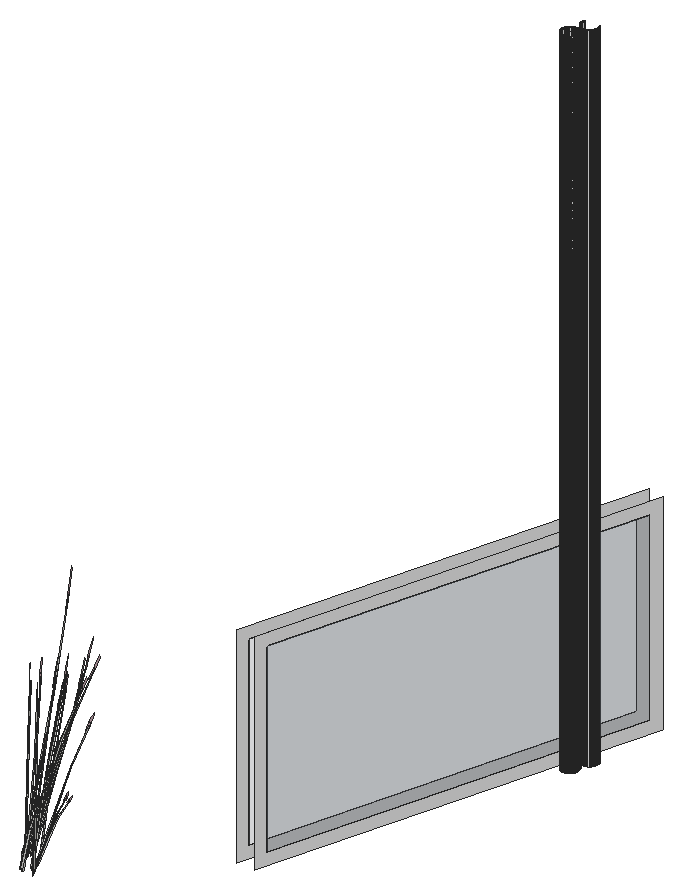
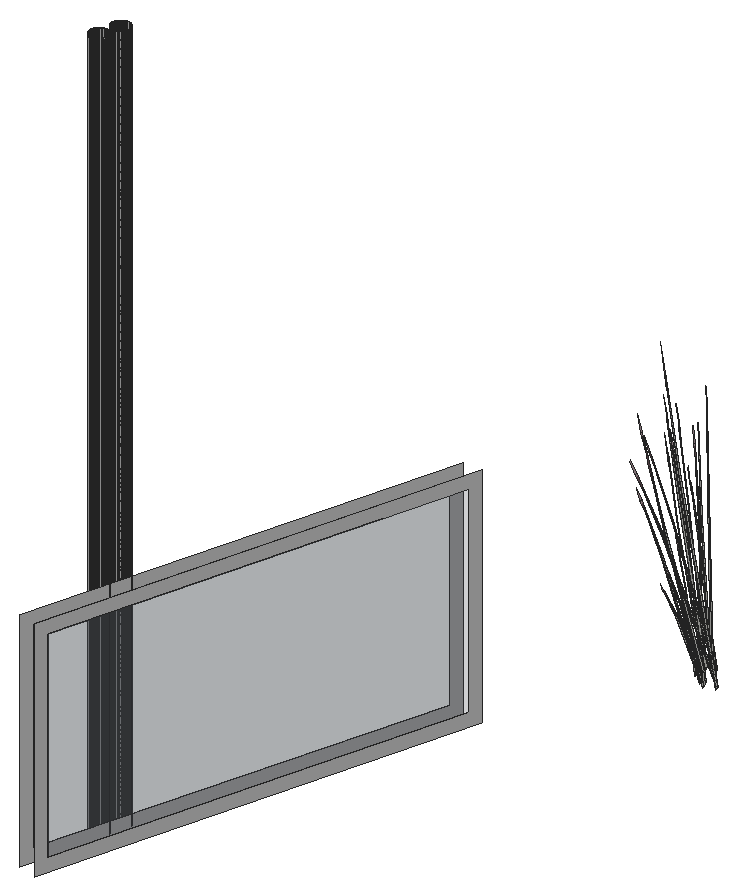
# SketchUp Ruby script. Lengths in inches.
U = 1.inch
M = Sketchup.active_model
def pt(a) = Geom::Point3d.new(a.map { |v| v * U })
def face(e, loops, mat)
  f = e.add_face(loops[0].map { |a| pt(a) })
  loops[1..].each { |l| e.add_face(l.map { |a| pt(a) }).erase! }
  f.material = f.back_material = mat if mat
  f
end
# faces: each face lists its corners as indices into pts; further lists are holes
def faces(e, pts, list, mat = nil) = list.each { |f| face(e, (f[0].is_a?(Array) ? f : [f]).map { |l| l.map { |i| pts[i] } }, mat) }
# xy, xz, yz: faces in a plane at the given z, y or x. An outline is a flat list of corners, or four numbers for a rectangle; further outlines are holes
def ring(l) = l.size == 4 ? [[l[0], l[1]], [l[2], l[1]], [l[2], l[3]], [l[0], l[3]]] : l.each_slice(2).to_a
def flat(e, list, mat, &to3) = list.each { |f| face(e, (f[0].is_a?(Array) ? f : [f]).map { |l| ring(l).map { |u, v| to3.(u, v) } }, mat) }
def xy(e, z, list, mat = nil) = flat(e, list, mat) { |x, y| [x, y, z] }
def xz(e, y, list, mat = nil) = flat(e, list, mat) { |x, z| [x, y, z] }
def yz(e, x, list, mat = nil) = flat(e, list, mat) { |y, z| [x, y, z] }
def lines(e, pts, list) = list.each { |a, b| e.add_line(pt(pts[a]), pt(pts[b])) }
# prism: a flat outline (further loops are holes) pulled along v
def prism(e, loops, v, mat = nil)
  f = face(e, loops, mat); d = Geom::Vector3d.new(v.map { |x| x * U })
  f.pushpull(f.normal.samedirection?(d) ? d.length : -d.length)
end
def box(e, o, s, mat = nil) = prism(e, [[o, [o[0] + s[0], o[1], o[2]], [o[0] + s[0], o[1] + s[1], o[2]], [o[0], o[1] + s[1], o[2]]]], [0, 0, s[2]], mat)
def at(x, y, z, deg = 0) = Geom::Transformation.translation(pt([x, y, z])) * Geom::Transformation.rotation(ORIGIN, Z_AXIS, deg.degrees)
def axes(o, x, y, z) = Geom::Transformation.new([*x, 0, *y, 0, *z, 0, *pt(o).to_a, 1])
def part(name) = M.definitions.add(name)
# library, detail: a bought-in or finely detailed component or shape, given as its bounding box
def library(name, o, s) = part(name).tap { |d| box(d.entities, o, s) }
def detail(e, o, s) = box(e.add_group.entities, o, s)
def put(e, d, t, mat = nil) = e.add_instance(d, t).tap { |i| i.material = mat if mat }
def group(e, t, mat = nil) = e.add_group.tap { |g| g.transformation = t; g.material = mat if mat }.entities
root = M.entities
M.materials.add("Glass_Basic_01").color = [105, 113, 122]
M.materials["Glass_Basic_01"].alpha = 0.25
M.materials.add("LightPink_Translucent").color = [144, 107, 117]
M.materials["LightPink_Translucent"].alpha = 0.75
M.materials.add("M01_Silver_Fog").color = [224, 224, 224]
c1 = part("blade")
p = [[2.15,0.21,22],[0,0.17,0],[0.09,0.45,0],[2.18,0.31,22],[2.29,0.31,22],[0.38,0.45,0],
  [2.48,0.24,33],[2.49,0.24,33],[2.48,0.22,33]]
faces(c1.entities,p,[[0,1,2,3],[4,5,2,3],[6,3,4,7],[8,0,3,6]])
c2 = part("seeds")
p = [[0.3,-0.1,1.38],[-0.01,-0.03,1.59],[-0.01,-0.03,0.03],[0.14,-0.07,-0.07],[0.29,-0.03,3],[0.15,0.01,3.11]]
faces(c2.entities,p,[[0,1,2,3],[1,0,4,5]],"LightPink_Translucent")
c3 = part("blade with seeds")
put(c3.entities,c1,at(0,0,0))
put(c3.entities,c2,axes([2.4,0.25,30.99],[1.5799,-0.05474,1.17369],[-0.12525,1.92788,0.29478],[-0.07173,-0.02425,1.56792]))
xz(root,421.6,[[358.82,522,358.91,636],[358.91,522,359,636]],"M01_Silver_Fog")
xz(root,421.95,[[359.74,522,359.83,636],[359.83,522,359.92,636]],"M01_Silver_Fog")
yz(root,357.51,[[420.11,522,420.2,636],[420.2,522,420.29,636]],"M01_Silver_Fog")
yz(root,358.43,[[423.26,522,423.35,636],[423.35,522,423.44,636]],"M01_Silver_Fog")
yz(root,360.31,[[420.11,522,420.2,636],[420.2,522,420.29,636]],"M01_Silver_Fog")
yz(root,361.23,[[423.26,522,423.35,636],[423.35,522,423.44,636]],"M01_Silver_Fog")
p = [[359.17,437.01,522],[340.07,371.78,522],[340.07,371.78,558],[359.17,437.01,558],[340.64,373.7,524],[358.6,435.09,524],
  [358.6,435.09,556],[340.64,373.7,556],[362.06,436.22,558],[343.2,371.78,558],[343.2,371.78,522],[362.06,436.22,522],
  [343.76,373.7,556],[361.5,434.3,556],[361.5,434.3,524],[343.76,373.7,524],[358.48,418.87,522],[358.5625,418.85,522],
  [358.5625,418.85,636],[358.48,418.87,636],[358.65,418.83,522],[358.73,418.8125,522],[358.73,418.8125,636],[358.65,418.83,636],
  [358.82,418.81,522],[358.82,418.81,636],[358.91,418.8,522],[358.91,418.8,636],[359,418.81,522],[359,418.81,636],
  [359.09,418.8125,522],[359.09,418.8125,636],[359.17,418.83,522],[359.17,418.83,636],[359.26,418.85,522],[359.26,418.85,636],
  [359.34,418.87,522],[359.34,418.87,636],[358.24,418.98,522],[358.3125,418.9375,522],[358.3125,418.9375,636],[358.24,418.98,636],
  [358.39,418.9,522],[358.39,418.9,636],[359.43,418.9,522],[359.43,418.9,636],[359.51,418.9375,522],[359.51,418.9375,636],
  [359.58,418.98,522],[359.58,418.98,636],[358.09,419.07,522],[358.16,419.02,522],[358.16,419.02,636],[358.09,419.07,636],
  [359.66,419.02,522],[359.66,419.02,636],[359.73,419.07,522],[359.73,419.07,636],[358.02,419.125,522],[358.02,419.125,636],
  [357.95,419.18,522],[357.95,419.18,636],[359.8,419.125,522],[359.8,419.125,636],[359.87,419.18,522],[359.87,419.18,636],
  [357.83,419.31,522],[357.89,419.24,522],[357.89,419.24,636],[357.83,419.31,636],[359.93,419.24,522],[359.93,419.24,636],
  [359.99,419.31,522],[359.99,419.31,636],[357.78,419.38,522],[357.78,419.38,636],[360.04,419.38,522],[360.04,419.38,636],
  [357.73,419.45,522],[357.73,419.45,636],[360.09,419.45,522],[360.09,419.45,636],[357.64,419.61,522],[357.68,419.53,522],
  [357.68,419.53,636],[357.64,419.61,636],[360.14,419.53,522],[360.14,419.53,636],[360.18,419.61,522],[360.18,419.61,636],
  [357.61,419.6875,522],[357.61,419.6875,636],[360.21,419.6875,522],[360.21,419.6875,636],[357.58,419.77,522],[357.58,419.77,636],
  [360.24,419.77,522],[360.24,419.77,636],[357.55,419.85,522],[357.55,419.85,636],[360.27,419.85,522],[360.27,419.85,636],
  [357.54,419.94,522],[357.54,419.94,636],[357.52,420.03,522],[357.52,420.03,636],[360.29,419.94,522],[360.29,419.94,636],
  [360.3,420.03,522],[360.3,420.03,636],[357.51,420.11,522],[357.51,420.11,636],[360.31,420.11,522],[360.31,420.11,636],
  [357.52,420.38,522],[357.51,420.29,522],[357.51,420.29,636],[357.52,420.38,636],[360.31,420.29,522],[360.3,420.38,522],
  [360.3,420.38,636],[360.31,420.29,636],[357.54,420.46,522],[357.54,420.46,636],[360.29,420.46,522],[360.29,420.46,636],
  [357.55,420.55,522],[357.55,420.55,636],[360.27,420.55,522],[360.27,420.55,636],[357.58,420.64,522],[357.58,420.64,636],
  [357.61,420.72,522],[357.61,420.72,636],[360.24,420.64,522],[360.24,420.64,636],[360.21,420.72,522],[360.21,420.72,636],
  [357.64,420.8,522],[357.64,420.8,636],[360.18,420.8,522],[360.18,420.8,636],[357.68,420.88,522],[357.68,420.88,636],
  [360.14,420.88,522],[360.14,420.88,636],[357.73,420.95,522],[357.73,420.95,636],[360.09,420.95,522],[360.09,420.95,636],
  [357.78,421.03,522],[357.78,421.03,636],[357.83,421.09,522],[357.83,421.09,636],[360.04,421.03,522],[360.04,421.03,636],
  [359.99,421.09,522],[359.99,421.09,636],[357.89,421.16,522],[357.89,421.16,636],[359.93,421.16,522],[359.93,421.16,636],
  [357.95,421.22,522],[357.95,421.22,636],[358.02,421.28,522],[358.02,421.28,636],[359.87,421.22,522],[359.8,421.28,522],
  [359.8,421.28,636],[359.87,421.22,636],[358.09,421.34,522],[358.09,421.34,636],[358.16,421.38,522],[358.16,421.38,636],
  [359.73,421.34,522],[359.73,421.34,636],[359.66,421.38,522],[359.66,421.38,636],[358.24,421.43,522],[358.24,421.43,636],
  [358.3125,421.47,522],[358.3125,421.47,636],[359.58,421.43,522],[359.51,421.47,522],[359.51,421.47,636],[359.58,421.43,636],
  [358.39,421.5,522],[358.39,421.5,636],[358.48,421.53,522],[358.48,421.53,636],[358.5625,421.56,522],[358.5625,421.56,636],
  [359.43,421.5,522],[359.34,421.53,522],[359.34,421.53,636],[359.43,421.5,636],[359.26,421.56,522],[359.26,421.56,636],
  [358.65,421.58,522],[358.65,421.58,636],[358.73,421.59,522],[358.73,421.59,636],[358.82,421.6,522],[358.82,421.6,636],
  [359.09,421.59,522],[359,421.6,522],[359,421.6,636],[359.09,421.59,636],[359.17,421.58,522],[359.17,421.58,636],
  [359.66,421.96,522],[359.74,421.95,522],[359.74,421.95,636],[359.66,421.96,636],[359.92,421.95,522],[360.01,421.96,522],
  [360.01,421.96,636],[359.92,421.95,636],[359.23,422.08,522],[359.32,422.05,522],[359.32,422.05,636],[359.23,422.08,636],
  [359.4,422.02,522],[359.4,422.02,636],[359.48,421.99,522],[359.48,421.99,636],[359.57,421.97,522],[359.57,421.97,636],
  [360.09,421.97,522],[360.09,421.97,636],[360.18,421.99,522],[360.18,421.99,636],[360.26,422.02,522],[360.26,422.02,636],
  [360.35,422.05,522],[360.35,422.05,636],[360.43,422.08,522],[360.43,422.08,636],[359.08,422.17,522],[359.16,422.12,522],
  [359.16,422.12,636],[359.08,422.17,636],[360.51,422.12,522],[360.51,422.12,636],[360.58,422.17,522],[360.58,422.17,636],
  [358.9375,422.27,522],[359.01,422.21,522],[359.01,422.21,636],[358.9375,422.27,636],[360.65,422.21,522],[360.65,422.21,636],
  [360.72,422.27,522],[360.72,422.27,636],[358.81,422.39,522],[358.87,422.33,522],[358.87,422.33,636],[358.81,422.39,636],
  [360.79,422.33,522],[360.79,422.33,636],[360.85,422.39,522],[360.85,422.39,636],[358.75,422.45,522],[358.75,422.45,636],
  [360.91,422.45,522],[360.91,422.45,636],[358.65,422.6,522],[358.7,422.52,522],[358.7,422.52,636],[358.65,422.6,636],
  [360.96,422.52,522],[360.96,422.52,636],[361.01,422.6,522],[361.01,422.6,636],[358.6,422.67,522],[358.6,422.67,636],
  [361.06,422.67,522],[361.06,422.67,636],[358.5625,422.75,522],[358.5625,422.75,636],[361.1,422.75,522],[361.1,422.75,636],
  [358.53,422.83,522],[358.53,422.83,636],[358.5,422.91,522],[358.5,422.91,636],[361.13,422.83,522],[361.13,422.83,636],
  [361.16,422.91,522],[361.16,422.91,636],[358.47,423,522],[358.47,423,636],[361.1875,423,522],[361.1875,423,636],
  [358.46,423.08,522],[358.46,423.08,636],[361.21,423.08,522],[361.21,423.08,636],[358.44,423.17,522],[358.44,423.17,636],
  [361.22,423.17,522],[361.22,423.17,636],[358.43,423.26,522],[358.43,423.26,636],[361.23,423.26,522],[361.23,423.26,636],
  [358.44,423.52,522],[358.43,423.44,522],[358.43,423.44,636],[358.44,423.52,636],[361.23,423.44,522],[361.22,423.52,522],
  [361.22,423.52,636],[361.23,423.44,636],[358.46,423.61,522],[358.46,423.61,636],[361.21,423.61,522],[361.21,423.61,636],
  [358.47,423.7,522],[358.47,423.7,636],[361.1875,423.7,522],[361.1875,423.7,636],[358.5,423.78,522],[358.5,423.78,636],
  [361.16,423.78,522],[361.16,423.78,636],[358.53,423.86,522],[358.53,423.86,636],[361.13,423.86,522],[361.13,423.86,636],
  [358.5625,423.94,522],[358.5625,423.94,636],[361.1,423.94,522],[361.1,423.94,636]]
faces(root,p,[[[0,1,2,3],[4,5,6,7]],[[8,9,10,11],[12,13,14,15]],[16,17,18,19],[20,21,22,23],[17,20,23,18],[21,24,25,22],[24,26,27,25],[26,28,29,27],
  [28,30,31,29],[30,32,33,31],[32,34,35,33],[34,36,37,35],[38,39,40,41],[39,42,43,40],[42,16,19,43],[36,44,45,37],
  [44,46,47,45],[46,48,49,47],[50,51,52,53],[51,38,41,52],[48,54,55,49],[54,56,57,55],[58,50,53,59],[60,58,59,61],
  [56,62,63,57],[62,64,65,63],[66,67,68,69],[67,60,61,68],[64,70,71,65],[70,72,73,71],[74,66,69,75],[72,76,77,73],
  [78,74,75,79],[76,80,81,77],[82,83,84,85],[83,78,79,84],[80,86,87,81],[86,88,89,87],[90,82,85,91],[88,92,93,89],
  [94,90,91,95],[92,96,97,93],[98,94,95,99],[96,100,101,97],[102,98,99,103],[104,102,103,105],[100,106,107,101],[106,108,109,107],
  [110,104,105,111],[108,112,113,109],[114,115,116,117],[118,119,120,121],[122,114,117,123],[119,124,125,120],[126,122,123,127],[124,128,129,125],
  [130,126,127,131],[132,130,131,133],[128,134,135,129],[134,136,137,135],[138,132,133,139],[136,140,141,137],[142,138,139,143],[140,144,145,141],
  [146,142,143,147],[144,148,149,145],[150,146,147,151],[152,150,151,153],[148,154,155,149],[154,156,157,155],[158,152,153,159],[156,160,161,157],
  [162,158,159,163],[164,162,163,165],[166,167,168,169],[160,166,169,161],[170,164,165,171],[172,170,171,173],[167,174,175,168],[174,176,177,175],
  [178,172,173,179],[180,178,179,181],[182,183,184,185],[176,182,185,177],[186,180,181,187],[188,186,187,189],[190,188,189,191],[192,193,194,195],
  [193,196,197,194],[183,192,195,184],[198,190,191,199],[200,198,199,201],[202,200,201,203],[204,205,206,207],[208,204,207,209],[196,208,209,197],
  [210,211,212,213],[214,215,216,217],[218,219,220,221],[219,222,223,220],[222,224,225,223],[224,226,227,225],[226,210,213,227],[215,228,229,216],
  [228,230,231,229],[230,232,233,231],[232,234,235,233],[234,236,237,235],[238,239,240,241],[239,218,221,240],[236,242,243,237],[242,244,245,243],
  [246,247,248,249],[247,238,241,248],[244,250,251,245],[250,252,253,251],[254,255,256,257],[255,246,249,256],[252,258,259,253],[258,260,261,259],
  [262,254,257,263],[260,264,265,261],[266,267,268,269],[267,262,263,268],[264,270,271,265],[270,272,273,271],[274,266,269,275],[272,276,277,273],
  [278,274,275,279],[276,280,281,277],[282,278,279,283],[284,282,283,285],[280,286,287,281],[286,288,289,287],[290,284,285,291],[288,292,293,289],
  [294,290,291,295],[292,296,297,293],[298,294,295,299],[296,300,301,297],[302,298,299,303],[300,304,305,301],[306,307,308,309],[310,311,312,313],
  [314,306,309,315],[311,316,317,312],[318,314,315,319],[316,320,321,317],[322,318,319,323],[320,324,325,321],[326,322,323,327],[324,328,329,325],
  [330,326,327,331],[328,332,333,329]],"M01_Silver_Fog")
faces(root,p,[[5,4,7,6],[13,12,15,14]],"Glass_Basic_01")
put(root,c3,axes([321.47,349.08,526.98],[0.26246,-0.42493,-0.71045],[0.45991,0.30199,0.08574],[0.15671,-0.15395,1.00501]))
put(root,c3,axes([321.85,348.69,524.59],[-0.1795,-0.01595,1.43002],[-0.18389,-0.42791,-0.30754],[0.22051,-0.12105,0.61141]))
put(root,c3,axes([322.06,347.91,524.77],[-0.16736,0.27414,1.1486],[-0.14385,-0.36832,0.84392],[0.13822,-0.09229,0.25299]))
put(root,c3,axes([321.82,348.9375,526.53],[0.43736,-0.07697,-0.35414],[0.11549,0.43998,0.4572],[0.12533,-0.11818,0.87481]))
put(root,c3,axes([321.68,349.98,526.68],[0.13612,-0.48987,-0.51099],[0.46669,0.16791,-0.3958],[0.1879,-0.04492,0.97773]))
put(root,c3,axes([322.18,350.12,523.98],[-0.32361,0.06463,1.41583],[-0.05151,-0.51444,0.08104],[0.22666,-0.07786,0.80566]))
put(root,c3,axes([322.77,349.66,524.26],[-0.31151,-0.34437,-0.06488],[0.34117,-0.31553,-0.29416],[0.09667,-0.02221,0.97024]))
put(root,c3,axes([321.59,350.16,526.98],[0.44151,-0.23785,-0.71045],[0.24605,0.4896,0.08574],[0.21333,-0.05562,1.00501]))
put(root,c3,axes([322.53,349.78,523.49],[-0.02626,-0.08176,1.76342],[0.18213,-0.47826,-0.26939],[0.18372,-0.00688,0.30037]))
put(root,c3,axes([321.97,350.2,526.53],[0.41757,0.15024,-0.35414],[-0.12179,0.4383,0.4572],[0.16812,-0.04019,0.87481]))
put(root,c3,axes([320.83,349.66,525.875],[-0.20841,0.0122,1.71376],[0.13825,-0.52864,0.13857],[0.297,0.0327,0.73262]))
put(root,c3,axes([320.55,349.34,524.06],[0.52267,0.08829,-0.62353],[-0.11029,0.54463,-0.16365],[0.15598,0.06599,1.37633]))
put(root,c3,axes([322.86,350.29,524.77],[-0.31044,0.08891,1.1486],[0.14613,-0.36744,0.84392],[0.16469,0.02514,0.25299]))
put(root,c3,axes([322.32,351.42,525.93],[-0.09617,-0.45271,-0.03492],[0.45453,-0.10408,-0.15832],[0.09492,0.0287,0.52218]))
put(root,c3,axes([322.27,350.88,524.59],[-0.12101,-0.13245,1.43002],[0.15744,-0.43816,-0.30754],[0.24483,0.05936,0.61141]))
put(root,c3,axes([321.16,351.15,526.98],[0.50227,0.01297,-0.71045],[-0.03373,0.54602,0.08574],[0.21278,0.05762,1.00501]))
put(root,c3,axes([321.46,351.37,526.53],[0.28589,0.33718,-0.35414],[-0.32644,0.31919,0.4572],[0.16586,0.04856,0.87481]))
put(root,c3,axes([320.4375,350.51,525.875],[-0.18664,-0.09279,1.71376],[0.38624,-0.38925,0.13857],[0.24072,0.1756,0.73262]))
